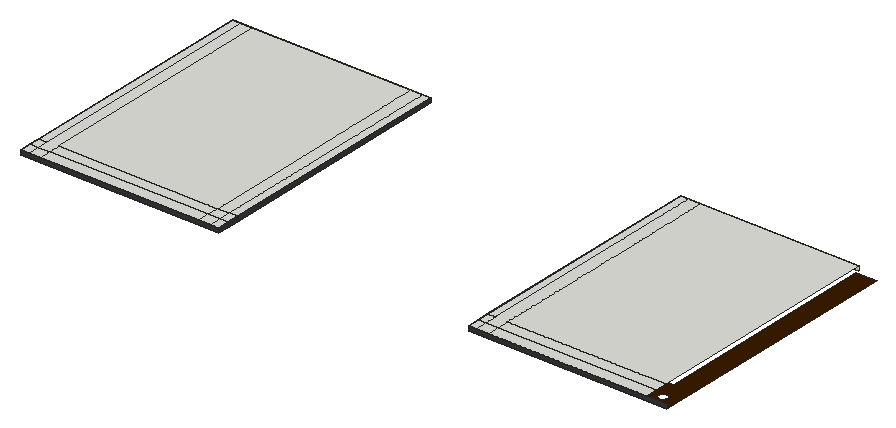
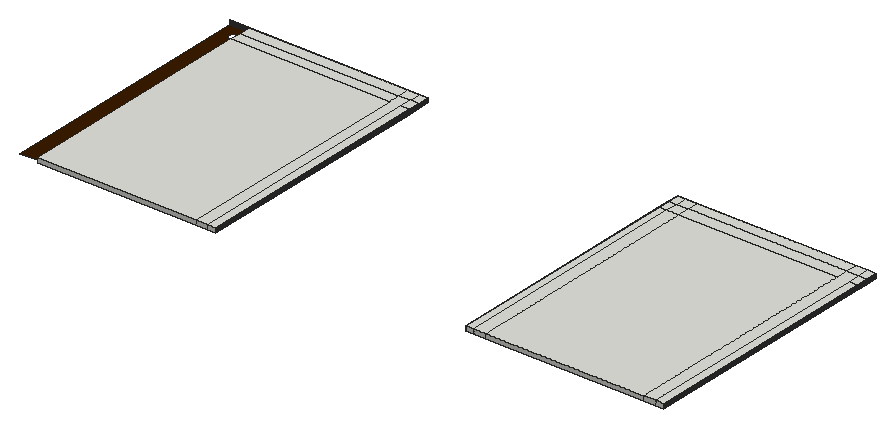
# SketchUp Ruby script. Lengths in inches.
U = 1.inch
M = Sketchup.active_model
def pt(a) = Geom::Point3d.new(a.map { |v| v * U })
def face(e, loops, mat)
  f = e.add_face(loops[0].map { |a| pt(a) })
  loops[1..].each { |l| e.add_face(l.map { |a| pt(a) }).erase! }
  f.material = f.back_material = mat if mat
  f
end
# faces: each face lists its corners as indices into pts; further lists are holes
def faces(e, pts, list, mat = nil) = list.each { |f| face(e, (f[0].is_a?(Array) ? f : [f]).map { |l| l.map { |i| pts[i] } }, mat) }
# xy, xz, yz: faces in a plane at the given z, y or x. An outline is a flat list of corners, or four numbers for a rectangle; further outlines are holes
def ring(l) = l.size == 4 ? [[l[0], l[1]], [l[2], l[1]], [l[2], l[3]], [l[0], l[3]]] : l.each_slice(2).to_a
def flat(e, list, mat, &to3) = list.each { |f| face(e, (f[0].is_a?(Array) ? f : [f]).map { |l| ring(l).map { |u, v| to3.(u, v) } }, mat) }
def xy(e, z, list, mat = nil) = flat(e, list, mat) { |x, y| [x, y, z] }
def xz(e, y, list, mat = nil) = flat(e, list, mat) { |x, z| [x, y, z] }
def yz(e, x, list, mat = nil) = flat(e, list, mat) { |y, z| [x, y, z] }
def lines(e, pts, list) = list.each { |a, b| e.add_line(pt(pts[a]), pt(pts[b])) }
# prism: a flat outline (further loops are holes) pulled along v
def prism(e, loops, v, mat = nil)
  f = face(e, loops, mat); d = Geom::Vector3d.new(v.map { |x| x * U })
  f.pushpull(f.normal.samedirection?(d) ? d.length : -d.length)
end
def box(e, o, s, mat = nil) = prism(e, [[o, [o[0] + s[0], o[1], o[2]], [o[0] + s[0], o[1] + s[1], o[2]], [o[0], o[1] + s[1], o[2]]]], [0, 0, s[2]], mat)
def at(x, y, z, deg = 0) = Geom::Transformation.translation(pt([x, y, z])) * Geom::Transformation.rotation(ORIGIN, Z_AXIS, deg.degrees)
def axes(o, x, y, z) = Geom::Transformation.new([*x, 0, *y, 0, *z, 0, *pt(o).to_a, 1])
def part(name) = M.definitions.add(name)
# library, detail: a bought-in or finely detailed component or shape, given as its bounding box
def library(name, o, s) = part(name).tap { |d| box(d.entities, o, s) }
def detail(e, o, s) = box(e.add_group.entities, o, s)
def put(e, d, t, mat = nil) = e.add_instance(d, t).tap { |i| i.material = mat if mat }
def group(e, t, mat = nil) = e.add_group.tap { |g| g.transformation = t; g.material = mat if mat }.entities
root = M.entities
M.materials.add("[Color C08]").color = [58, 29, 0]
M.materials.add("[Color M07]").color = [58, 58, 58]
xy(root,502.5625,[[86.0625,283.04,285.28,283.04,285.28,362.98,280.83,362.98,280.83,287.65,90.67,287.65,90.67,570.3125,285.28,570.3125,285.28,574.92,86.0625,574.92],[90.67,287.65,90.67,570.3125,285.28,570.3125,285.28,362.98,280.83,362.98,280.83,287.65],[285.28,570.3125,300.28,574.92],[300.28,570.3125,310.47,574.92]])
xy(root,502.5625,[[[60.9375,241.85,60.9375,574.92,86.0625,574.92,86.0625,283.04,285.28,283.04,285.28,570.3125,310.47,570.3125,310.47,241.85],[205.83,251.93,207.38,252.13,208.83,252.72,210.08,253.67,211.04,254.91,211.64,256.36,211.85,257.91,211.65,259.46,211.05,260.91,210.1,262.16,208.86,263.12,207.42,263.72,205.87,263.93,204.3125,263.73,202.86,263.13,201.62,262.18,200.66,260.94,200.06,259.5,199.85,257.95,200.05,256.39,200.64,254.94,201.59,253.7,202.83,252.74,204.28,252.14],[87.64,251.93,89.2,252.13,90.65,252.72,91.89,253.67,92.85,254.91,93.45,256.36,93.66,257.91,93.46,259.46,92.87,260.91,91.92,262.16,90.68,263.12,89.23,263.72,87.68,263.93,86.125,263.73,84.68,263.13,83.43,262.18,82.47,260.94,81.87,259.5,81.66,257.95,81.86,256.39,82.46,254.94,83.41,253.7,84.65,252.74,86.09,252.14],[155.02,251.93,156.57,252.13,158.02,252.72,159.27,253.67,160.22,254.91,160.83,256.36,161.04,257.91,160.84,259.46,160.24,260.91,159.29,262.16,158.05,263.12,156.61,263.72,155.05,263.93,153.5,263.73,152.05,263.13,150.81,262.18,149.85,260.94,149.25,259.5,149.04,257.95,149.24,256.39,149.83,254.94,150.78,253.7,152.02,252.74,153.47,252.14],[253.08,251.93,254.63,252.13,256.08,252.72,257.33,253.67,258.29,254.91,258.89,256.36,259.1,257.91,258.9,259.46,258.3,260.91,257.35,262.16,256.11,263.12,254.67,263.72,253.12,263.93,251.5625,263.73,250.11,263.13,248.87,262.18,247.91,260.94,247.31,259.5,247.1,257.95,247.3,256.39,247.89,254.94,248.84,253.7,250.08,252.74,251.53,252.14],[292.46,251.93,294.01,252.13,295.46,252.72,296.7,253.67,297.66,254.91,298.26,256.36,298.47,257.91,298.27,259.46,297.68,260.91,296.73,262.16,295.49,263.12,294.04,263.72,292.49,263.93,290.9375,263.73,289.49,263.13,288.24,262.18,287.29,260.94,286.68,259.5,286.47,257.95,286.67,256.39,287.27,254.94,288.22,253.7,289.46,252.74,290.9,252.14]],[[624.0625,241.85,624.0625,574.92,649.1875,574.92,649.1875,283.04,848.4,283.04,848.4,570.3125,873.59,570.3125,873.59,241.85],[768.96,251.93,770.51,252.13,771.96,252.72,773.2,253.67,774.16,254.91,774.76,256.36,774.97,257.91,774.77,259.46,774.18,260.91,773.23,262.16,771.99,263.12,770.54,263.72,768.99,263.93,767.4375,263.73,765.99,263.13,764.74,262.18,763.79,260.94,763.18,259.5,762.97,257.95,763.17,256.39,763.77,254.94,764.72,253.7,765.96,252.74,767.4,252.14],[650.77,251.93,652.32,252.13,653.77,252.72,655.02,253.67,655.97,254.91,656.58,256.36,656.79,257.91,656.59,259.46,655.99,260.91,655.04,262.16,653.8,263.12,652.36,263.72,650.8,263.93,649.25,263.73,647.8,263.13,646.56,262.18,645.6,260.94,645,259.5,644.79,257.95,644.99,256.39,645.58,254.94,646.53,253.7,647.77,252.74,649.22,252.14],[718.14,251.93,719.7,252.13,721.15,252.72,722.39,253.67,723.35,254.91,723.95,256.36,724.16,257.91,723.96,259.46,723.37,260.91,722.42,262.16,721.18,263.12,719.73,263.72,718.18,263.93,716.625,263.73,715.18,263.13,713.93,262.18,712.97,260.94,712.37,259.5,712.16,257.95,712.36,256.39,712.96,254.94,713.91,253.7,715.15,252.74,716.59,252.14],[816.21,251.93,817.76,252.13,819.21,252.72,820.45,253.67,821.41,254.91,822.01,256.36,822.22,257.91,822.02,259.46,821.43,260.91,820.48,262.16,819.24,263.12,817.79,263.72,816.24,263.93,814.6875,263.73,813.24,263.13,811.99,262.18,811.04,260.94,810.43,259.5,810.22,257.95,810.42,256.39,811.02,254.94,811.97,253.7,813.21,252.74,814.65,252.14],[855.58,251.93,857.13,252.13,858.58,252.72,859.83,253.67,860.79,254.91,861.39,256.36,861.6,257.91,861.4,259.46,860.8,260.91,859.85,262.16,858.61,263.12,857.17,263.72,855.62,263.93,854.0625,263.73,852.61,263.13,851.37,262.18,850.41,260.94,849.81,259.5,849.6,257.95,849.8,256.39,850.39,254.94,851.34,253.7,852.58,252.74,854.03,252.14]]],"[Color C08]")
xy(root,503.4375,[[87.64,251.93,86.09,252.14,84.65,252.74,83.41,253.7,82.46,254.94,81.86,256.39,81.66,257.95,81.87,259.5,82.47,260.94,83.43,262.18,84.68,263.13,86.125,263.73,87.68,263.93,89.23,263.72,90.68,263.12,91.92,262.16,92.87,260.91,93.46,259.46,93.66,257.91,93.45,256.36,92.85,254.91,91.89,253.67,90.65,252.72,89.2,252.13],[155.02,251.93,153.47,252.14,152.02,252.74,150.78,253.7,149.83,254.94,149.24,256.39,149.04,257.95,149.25,259.5,149.85,260.94,150.81,262.18,152.05,263.13,153.5,263.73,155.05,263.93,156.61,263.72,158.05,263.12,159.29,262.16,160.24,260.91,160.84,259.46,161.04,257.91,160.83,256.36,160.22,254.91,159.27,253.67,158.02,252.72,156.57,252.13],[205.83,251.93,204.28,252.14,202.83,252.74,201.59,253.7,200.64,254.94,200.05,256.39,199.85,257.95,200.06,259.5,200.66,260.94,201.62,262.18,202.86,263.13,204.3125,263.73,205.87,263.93,207.42,263.72,208.86,263.12,210.1,262.16,211.05,260.91,211.65,259.46,211.85,257.91,211.64,256.36,211.04,254.91,210.08,253.67,208.83,252.72,207.38,252.13],[253.08,251.93,251.53,252.14,250.08,252.74,248.84,253.7,247.89,254.94,247.3,256.39,247.1,257.95,247.31,259.5,247.91,260.94,248.87,262.18,250.11,263.13,251.5625,263.73,253.12,263.93,254.67,263.72,256.11,263.12,257.35,262.16,258.3,260.91,258.9,259.46,259.1,257.91,258.89,256.36,258.29,254.91,257.33,253.67,256.08,252.72,254.63,252.13],[292.46,251.93,290.9,252.14,289.46,252.74,288.22,253.7,287.27,254.94,286.67,256.39,286.47,257.95,286.68,259.5,287.29,260.94,288.24,262.18,289.49,263.13,290.9375,263.73,292.49,263.93,294.04,263.72,295.49,263.12,296.73,262.16,297.68,260.91,298.27,259.46,298.47,257.91,298.26,256.36,297.66,254.91,296.7,253.67,295.46,252.72,294.01,252.13],
  [650.77,251.93,649.22,252.14,647.77,252.74,646.53,253.7,645.58,254.94,644.99,256.39,644.79,257.95,645,259.5,645.6,260.94,646.56,262.18,647.8,263.13,649.25,263.73,650.8,263.93,652.36,263.72,653.8,263.12,655.04,262.16,655.99,260.91,656.59,259.46,656.79,257.91,656.58,256.36,655.97,254.91,655.02,253.67,653.77,252.72,652.32,252.13],[718.14,251.93,716.59,252.14,715.15,252.74,713.91,253.7,712.96,254.94,712.36,256.39,712.16,257.95,712.37,259.5,712.97,260.94,713.93,262.18,715.18,263.13,716.625,263.73,718.18,263.93,719.73,263.72,721.18,263.12,722.42,262.16,723.37,260.91,723.96,259.46,724.16,257.91,723.95,256.36,723.35,254.91,722.39,253.67,721.15,252.72,719.7,252.13]])
xy(root,508.5625,[[60.9375,241.85,71.125,256.29],[71.125,241.85,86.0625,256.29],[86.0625,241.85,285.28,256.29],[285.28,241.85,300.28,256.29],[300.28,241.85,310.47,256.29],
  [624.0625,241.85,634.25,256.29],[634.25,241.85,649.1875,256.29],[649.1875,241.85,848.4,256.29],[60.9375,256.29,71.125,271.23],[71.125,256.29,86.0625,574.92],
  [86.0625,256.29,285.28,271.23],[285.28,256.29,300.28,271.23],[300.28,256.29,310.47,271.23],[624.0625,256.29,634.25,271.23],[634.25,256.29,649.1875,574.92],
  [649.1875,256.29,848.4,271.23],[60.9375,271.23,71.125,574.92],[86.0625,271.23,285.28,574.92],[285.28,271.23,300.28,574.92],[300.28,271.23,310.47,574.92],
  [624.0625,271.23,634.25,574.92],[649.1875,271.23,848.4,574.92]])
xz(root,241.85,[[60.9375,502.5625,310.47,508.5625],[624.0625,502.5625,873.59,508.5625]],"[Color M07]")
xz(root,574.92,[[60.9375,502.5625,71.125,508.5625],[71.125,502.5625,86.0625,508.5625],[86.0625,502.5625,285.28,508.5625],[285.28,502.5625,300.28,508.5625],[300.28,502.5625,310.47,508.5625],
  [624.0625,502.5625,634.25,508.5625],[634.25,502.5625,649.1875,508.5625],[649.1875,502.5625,848.4,508.5625]])
yz(root,60.9375,[[241.85,502.5625,256.29,508.5625],[256.29,502.5625,271.23,508.5625],[271.23,502.5625,574.92,508.5625]],"[Color M07]")
yz(root,310.47,[[241.85,502.5625,256.29,508.5625],[256.29,502.5625,271.23,508.5625],[271.23,502.5625,574.92,508.5625]],"[Color M07]")
yz(root,624.0625,[[241.85,502.5625,256.29,508.5625],[256.29,502.5625,271.23,508.5625],[271.23,502.5625,574.92,508.5625]],"[Color M07]")
p = [[87.64,251.93,502.5625],[86.09,252.14,502.5625],[86.09,252.14,503.4375],[87.64,251.93,503.4375],[89.2,252.13,502.5625],[89.2,252.13,503.4375],
  [155.02,251.93,502.5625],[153.47,252.14,502.5625],[153.47,252.14,503.4375],[155.02,251.93,503.4375],[156.57,252.13,502.5625],[156.57,252.13,503.4375],
  [205.83,251.93,502.5625],[204.28,252.14,502.5625],[204.28,252.14,503.4375],[205.83,251.93,503.4375],[207.38,252.13,502.5625],[207.38,252.13,503.4375],
  [253.08,251.93,502.5625],[251.53,252.14,502.5625],[251.53,252.14,503.4375],[253.08,251.93,503.4375],[254.63,252.13,502.5625],[254.63,252.13,503.4375],
  [292.46,251.93,502.5625],[290.9,252.14,502.5625],[290.9,252.14,503.4375],[292.46,251.93,503.4375],[294.01,252.13,502.5625],[294.01,252.13,503.4375],
  [650.77,251.93,502.5625],[649.22,252.14,502.5625],[649.22,252.14,503.4375],[650.77,251.93,503.4375],[652.32,252.13,502.5625],[652.32,252.13,503.4375],
  [718.14,251.93,502.5625],[716.59,252.14,502.5625],[716.59,252.14,503.4375],[718.14,251.93,503.4375],[719.7,252.13,502.5625],[719.7,252.13,503.4375],
  [768.96,251.93,502.5625],[767.4,252.14,502.5625],[767.4,252.14,503.4375],[768.96,251.93,503.4375],[84.65,252.74,502.5625],[84.65,252.74,503.4375],
  [90.65,252.72,502.5625],[90.65,252.72,503.4375],[152.02,252.74,502.5625],[152.02,252.74,503.4375],[158.02,252.72,502.5625],[158.02,252.72,503.4375],
  [202.83,252.74,502.5625],[202.83,252.74,503.4375],[208.83,252.72,502.5625],[208.83,252.72,503.4375],[250.08,252.74,502.5625],[250.08,252.74,503.4375],
  [256.08,252.72,502.5625],[256.08,252.72,503.4375],[289.46,252.74,502.5625],[289.46,252.74,503.4375],[295.46,252.72,502.5625],[295.46,252.72,503.4375],
  [647.77,252.74,502.5625],[647.77,252.74,503.4375],[653.77,252.72,502.5625],[653.77,252.72,503.4375],[715.15,252.74,502.5625],[715.15,252.74,503.4375],
  [721.15,252.72,502.5625],[721.15,252.72,503.4375],[765.96,252.74,502.5625],[765.96,252.74,503.4375],[83.41,253.7,502.5625],[83.41,253.7,503.4375],
  [91.89,253.67,502.5625],[91.89,253.67,503.4375],[150.78,253.7,502.5625],[150.78,253.7,503.4375],[159.27,253.67,502.5625],[159.27,253.67,503.4375],
  [201.59,253.7,502.5625],[201.59,253.7,503.4375],[210.08,253.67,502.5625],[210.08,253.67,503.4375],[248.84,253.7,502.5625],[248.84,253.7,503.4375],
  [257.33,253.67,502.5625],[257.33,253.67,503.4375],[288.22,253.7,502.5625],[288.22,253.7,503.4375],[296.7,253.67,502.5625],[296.7,253.67,503.4375],
  [646.53,253.7,502.5625],[646.53,253.7,503.4375],[655.02,253.67,502.5625],[655.02,253.67,503.4375],[713.91,253.7,502.5625],[713.91,253.7,503.4375],
  [722.39,253.67,502.5625],[722.39,253.67,503.4375],[764.72,253.7,502.5625],[764.72,253.7,503.4375],[82.46,254.94,502.5625],[82.46,254.94,503.4375],
  [92.85,254.91,502.5625],[92.85,254.91,503.4375],[149.83,254.94,502.5625],[149.83,254.94,503.4375],[160.22,254.91,502.5625],[160.22,254.91,503.4375],
  [200.64,254.94,502.5625],[200.64,254.94,503.4375],[211.04,254.91,502.5625],[211.04,254.91,503.4375],[247.89,254.94,502.5625],[247.89,254.94,503.4375],
  [258.29,254.91,502.5625],[258.29,254.91,503.4375],[287.27,254.94,502.5625],[287.27,254.94,503.4375],[297.66,254.91,502.5625],[297.66,254.91,503.4375],
  [645.58,254.94,502.5625],[645.58,254.94,503.4375],[655.97,254.91,502.5625],[655.97,254.91,503.4375],[712.96,254.94,502.5625],[712.96,254.94,503.4375],
  [723.35,254.91,502.5625],[723.35,254.91,503.4375],[763.77,254.94,502.5625],[763.77,254.94,503.4375],[81.86,256.39,502.5625],[81.86,256.39,503.4375],
  [93.45,256.36,502.5625],[93.45,256.36,503.4375],[149.24,256.39,502.5625],[149.24,256.39,503.4375],[160.83,256.36,502.5625],[160.83,256.36,503.4375],
  [200.05,256.39,502.5625],[200.05,256.39,503.4375],[211.64,256.36,502.5625],[211.64,256.36,503.4375],[247.3,256.39,502.5625],[247.3,256.39,503.4375],
  [258.89,256.36,502.5625],[258.89,256.36,503.4375],[286.67,256.39,502.5625],[286.67,256.39,503.4375],[298.26,256.36,502.5625],[298.26,256.36,503.4375],
  [644.99,256.39,502.5625],[644.99,256.39,503.4375],[656.58,256.36,502.5625],[656.58,256.36,503.4375],[712.36,256.39,502.5625],[712.36,256.39,503.4375],
  [723.95,256.36,502.5625],[723.95,256.36,503.4375],[763.17,256.39,502.5625],[763.17,256.39,503.4375],[81.66,257.95,502.5625],[81.66,257.95,503.4375],
  [93.66,257.91,502.5625],[93.66,257.91,503.4375],[149.04,257.95,502.5625],[149.04,257.95,503.4375],[161.04,257.91,502.5625],[161.04,257.91,503.4375],
  [199.85,257.95,502.5625],[199.85,257.95,503.4375],[211.85,257.91,502.5625],[211.85,257.91,503.4375],[247.1,257.95,502.5625],[247.1,257.95,503.4375],
  [259.1,257.91,502.5625],[259.1,257.91,503.4375],[286.47,257.95,502.5625],[286.47,257.95,503.4375],[298.47,257.91,502.5625],[298.47,257.91,503.4375],
  [644.79,257.95,502.5625],[644.79,257.95,503.4375],[656.79,257.91,502.5625],[656.79,257.91,503.4375],[712.16,257.95,502.5625],[712.16,257.95,503.4375],
  [724.16,257.91,502.5625],[724.16,257.91,503.4375],[762.97,257.95,502.5625],[762.97,257.95,503.4375],[81.87,259.5,502.5625],[81.87,259.5,503.4375],
  [93.46,259.46,502.5625],[93.46,259.46,503.4375],[149.25,259.5,502.5625],[149.25,259.5,503.4375],[160.84,259.46,502.5625],[160.84,259.46,503.4375],
  [200.06,259.5,502.5625],[200.06,259.5,503.4375],[211.65,259.46,502.5625],[211.65,259.46,503.4375],[247.31,259.5,502.5625],[247.31,259.5,503.4375],
  [258.9,259.46,502.5625],[258.9,259.46,503.4375],[286.68,259.5,502.5625],[286.68,259.5,503.4375],[298.27,259.46,502.5625],[298.27,259.46,503.4375],
  [645,259.5,502.5625],[645,259.5,503.4375],[656.59,259.46,502.5625],[656.59,259.46,503.4375],[712.37,259.5,502.5625],[712.37,259.5,503.4375],
  [723.96,259.46,502.5625],[723.96,259.46,503.4375],[763.18,259.5,502.5625],[763.18,259.5,503.4375],[82.47,260.94,502.5625],[82.47,260.94,503.4375],
  [92.87,260.91,502.5625],[92.87,260.91,503.4375],[149.85,260.94,502.5625],[149.85,260.94,503.4375],[160.24,260.91,502.5625],[160.24,260.91,503.4375],
  [200.66,260.94,502.5625],[200.66,260.94,503.4375],[211.05,260.91,502.5625],[211.05,260.91,503.4375],[247.91,260.94,502.5625],[247.91,260.94,503.4375],
  [258.3,260.91,502.5625],[258.3,260.91,503.4375],[287.29,260.94,502.5625],[287.29,260.94,503.4375],[297.68,260.91,502.5625],[297.68,260.91,503.4375],
  [645.6,260.94,502.5625],[645.6,260.94,503.4375],[655.99,260.91,502.5625],[655.99,260.91,503.4375],[712.97,260.94,502.5625],[712.97,260.94,503.4375],
  [723.37,260.91,502.5625],[723.37,260.91,503.4375],[763.79,260.94,502.5625],[763.79,260.94,503.4375],[83.43,262.18,502.5625],[83.43,262.18,503.4375],
  [91.92,262.16,502.5625],[91.92,262.16,503.4375],[150.81,262.18,502.5625],[150.81,262.18,503.4375],[159.29,262.16,502.5625],[159.29,262.16,503.4375],
  [201.62,262.18,502.5625],[201.62,262.18,503.4375],[210.1,262.16,502.5625],[210.1,262.16,503.4375],[248.87,262.18,502.5625],[248.87,262.18,503.4375],
  [257.35,262.16,502.5625],[257.35,262.16,503.4375],[288.24,262.18,502.5625],[288.24,262.18,503.4375],[296.73,262.16,502.5625],[296.73,262.16,503.4375],
  [646.56,262.18,502.5625],[646.56,262.18,503.4375],[655.04,262.16,502.5625],[655.04,262.16,503.4375],[713.93,262.18,502.5625],[713.93,262.18,503.4375],
  [722.42,262.16,502.5625],[722.42,262.16,503.4375],[764.74,262.18,502.5625],[764.74,262.18,503.4375],[84.68,263.13,502.5625],[84.68,263.13,503.4375],
  [90.68,263.12,502.5625],[90.68,263.12,503.4375],[152.05,263.13,502.5625],[152.05,263.13,503.4375],[158.05,263.12,502.5625],[158.05,263.12,503.4375],
  [202.86,263.13,502.5625],[202.86,263.13,503.4375],[208.86,263.12,502.5625],[208.86,263.12,503.4375],[250.11,263.13,502.5625],[250.11,263.13,503.4375],
  [256.11,263.12,502.5625],[256.11,263.12,503.4375],[289.49,263.13,502.5625],[289.49,263.13,503.4375],[295.49,263.12,502.5625],[295.49,263.12,503.4375],
  [647.8,263.13,502.5625],[647.8,263.13,503.4375],[653.8,263.12,502.5625],[653.8,263.12,503.4375],[715.18,263.13,502.5625],[715.18,263.13,503.4375],
  [721.18,263.12,502.5625],[721.18,263.12,503.4375],[765.99,263.13,502.5625],[765.99,263.13,503.4375],[86.125,263.73,502.5625],[86.125,263.73,503.4375],
  [89.23,263.72,502.5625],[89.23,263.72,503.4375],[153.5,263.73,502.5625],[153.5,263.73,503.4375],[156.61,263.72,502.5625],[156.61,263.72,503.4375],
  [204.3125,263.73,502.5625],[204.3125,263.73,503.4375],[207.42,263.72,502.5625],[207.42,263.72,503.4375],[251.5625,263.73,502.5625],[251.5625,263.73,503.4375],
  [254.67,263.72,502.5625],[254.67,263.72,503.4375],[290.9375,263.73,502.5625],[290.9375,263.73,503.4375],[294.04,263.72,502.5625],[294.04,263.72,503.4375],
  [649.25,263.73,502.5625],[649.25,263.73,503.4375],[652.36,263.72,502.5625],[652.36,263.72,503.4375],[716.625,263.73,502.5625],[716.625,263.73,503.4375],
  [719.73,263.72,502.5625],[719.73,263.72,503.4375],[767.4375,263.73,502.5625],[767.4375,263.73,503.4375],[87.68,263.93,502.5625],[87.68,263.93,503.4375],
  [155.05,263.93,502.5625],[155.05,263.93,503.4375],[205.87,263.93,502.5625],[205.87,263.93,503.4375],[253.12,263.93,502.5625],[253.12,263.93,503.4375],
  [292.49,263.93,502.5625],[292.49,263.93,503.4375],[650.8,263.93,502.5625],[650.8,263.93,503.4375],[718.18,263.93,502.5625],[718.18,263.93,503.4375],
  [768.99,263.93,502.5625],[768.99,263.93,503.4375],[649.1875,256.29,502.5625],[649.1875,256.29,508.5625],[634.25,256.29,502.5625],[634.25,256.29,508.5625],
  [71.125,256.29,502.5625],[71.125,256.29,508.5625],[86.0625,256.29,502.5625],[86.0625,256.29,508.5625]]
faces(root,p,[[0,1,2,3],[4,0,3,5],[6,7,8,9],[10,6,9,11],[12,13,14,15],[16,12,15,17],[18,19,20,21],[22,18,21,23],
  [24,25,26,27],[28,24,27,29],[30,31,32,33],[34,30,33,35],[36,37,38,39],[40,36,39,41],[42,43,44,45],[1,46,47,2],
  [48,4,5,49],[7,50,51,8],[52,10,11,53],[13,54,55,14],[56,16,17,57],[19,58,59,20],[60,22,23,61],[25,62,63,26],
  [64,28,29,65],[31,66,67,32],[68,34,35,69],[37,70,71,38],[72,40,41,73],[43,74,75,44],[46,76,77,47],[78,48,49,79],
  [50,80,81,51],[82,52,53,83],[54,84,85,55],[86,56,57,87],[58,88,89,59],[90,60,61,91],[62,92,93,63],[94,64,65,95],
  [66,96,97,67],[98,68,69,99],[70,100,101,71],[102,72,73,103],[74,104,105,75],[76,106,107,77],[108,78,79,109],[80,110,111,81],
  [112,82,83,113],[84,114,115,85],[116,86,87,117],[88,118,119,89],[120,90,91,121],[92,122,123,93],[124,94,95,125],[96,126,127,97],
  [128,98,99,129],[100,130,131,101],[132,102,103,133],[104,134,135,105],[106,136,137,107],[138,108,109,139],[110,140,141,111],[142,112,113,143],
  [114,144,145,115],[146,116,117,147],[118,148,149,119],[150,120,121,151],[122,152,153,123],[154,124,125,155],[126,156,157,127],[158,128,129,159],
  [130,160,161,131],[162,132,133,163],[134,164,165,135],[136,166,167,137],[168,138,139,169],[140,170,171,141],[172,142,143,173],[144,174,175,145],
  [176,146,147,177],[148,178,179,149],[180,150,151,181],[152,182,183,153],[184,154,155,185],[156,186,187,157],[188,158,159,189],[160,190,191,161],
  [192,162,163,193],[164,194,195,165],[166,196,197,167],[198,168,169,199],[170,200,201,171],[202,172,173,203],[174,204,205,175],[206,176,177,207],
  [178,208,209,179],[210,180,181,211],[182,212,213,183],[214,184,185,215],[186,216,217,187],[218,188,189,219],[190,220,221,191],[222,192,193,223],
  [194,224,225,195],[196,226,227,197],[228,198,199,229],[200,230,231,201],[232,202,203,233],[204,234,235,205],[236,206,207,237],[208,238,239,209],
  [240,210,211,241],[212,242,243,213],[244,214,215,245],[216,246,247,217],[248,218,219,249],[220,250,251,221],[252,222,223,253],[224,254,255,225],
  [226,256,257,227],[258,228,229,259],[230,260,261,231],[262,232,233,263],[234,264,265,235],[266,236,237,267],[238,268,269,239],[270,240,241,271],
  [242,272,273,243],[274,244,245,275],[246,276,277,247],[278,248,249,279],[250,280,281,251],[282,252,253,283],[254,284,285,255],[256,286,287,257],
  [288,258,259,289],[260,290,291,261],[292,262,263,293],[264,294,295,265],[296,266,267,297],[268,298,299,269],[300,270,271,301],[272,302,303,273],
  [304,274,275,305],[276,306,307,277],[308,278,279,309],[280,310,311,281],[312,282,283,313],[284,314,315,285],[286,316,317,287],[318,288,289,319],
  [290,320,321,291],[322,292,293,323],[294,324,325,295],[326,296,297,327],[298,328,329,299],[330,300,301,331],[302,332,333,303],[334,304,305,335],
  [306,336,337,307],[338,308,309,339],[310,340,341,311],[342,312,313,343],[314,344,345,315],[316,346,347,317],[346,318,319,347],[320,348,349,321],
  [348,322,323,349],[324,350,351,325],[350,326,327,351],[328,352,353,329],[352,330,331,353],[332,354,355,333],[354,334,335,355],[336,356,357,337],
  [356,338,339,357],[340,358,359,341],[358,342,343,359],[344,360,361,345]])
lines(root,p,[[362,363],[364,365],[366,367],[368,369]])
